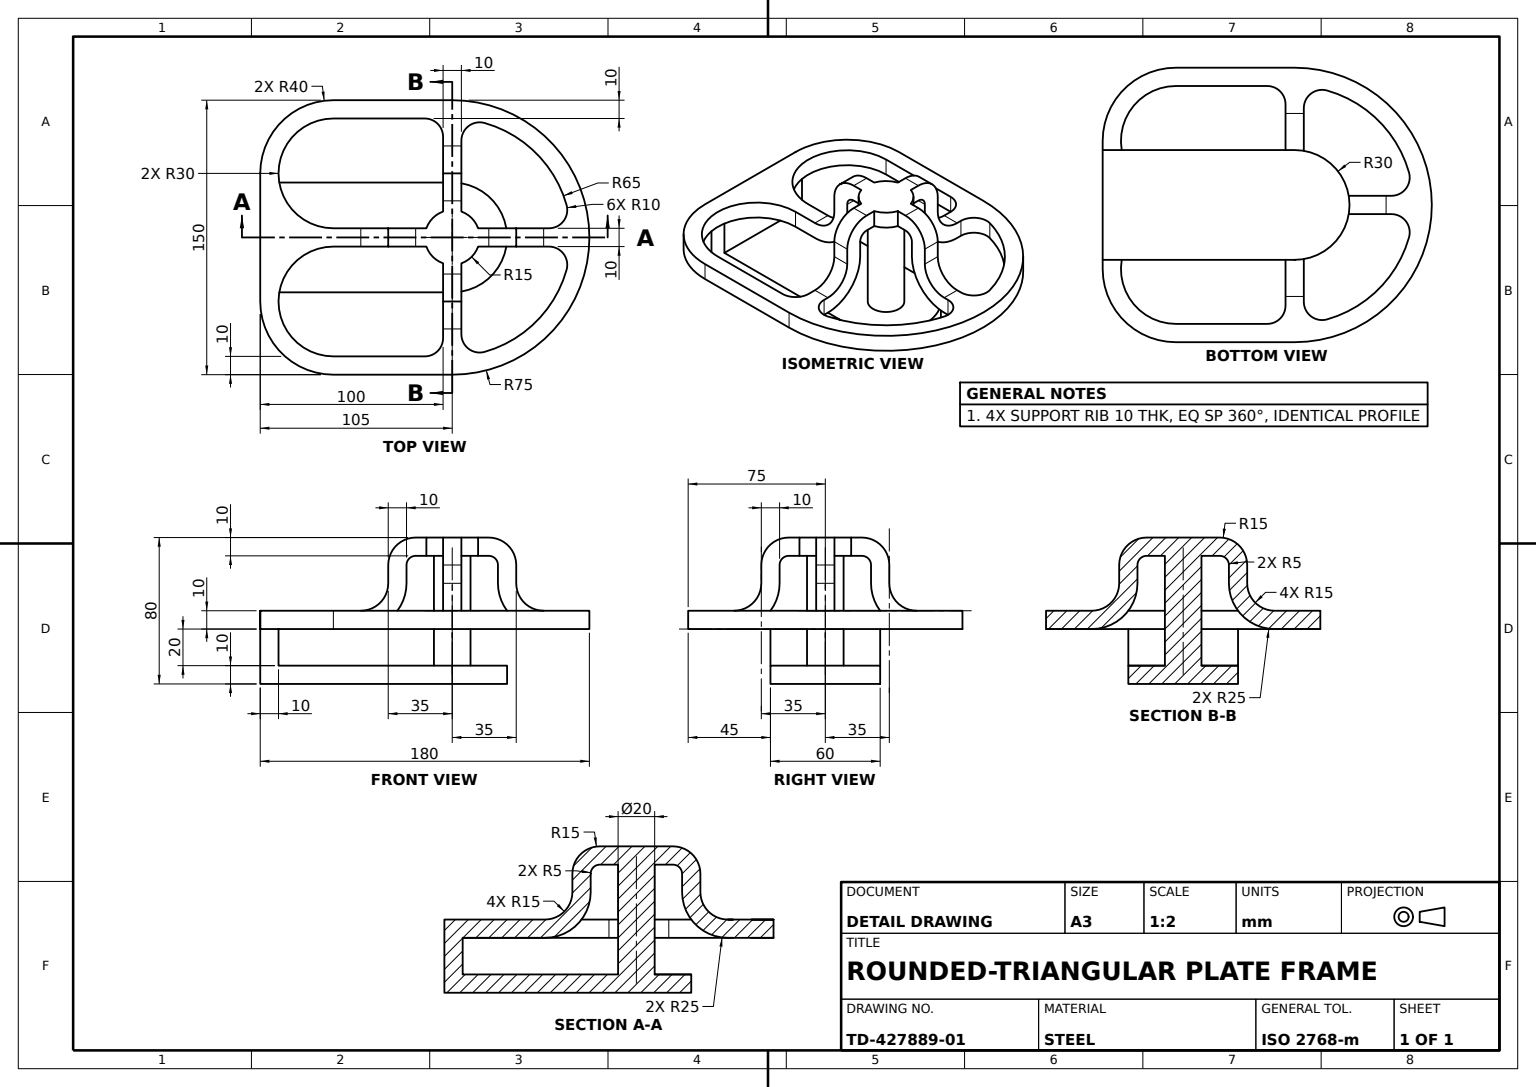
solid
v1 (-95,-30,30)
v2 (-95,-10,30)
e1 v1 v2 LINE
v3 (-105,-10,30)
e2 v2 v3 LINE
v4 (-105,-40,30)
e3 v3 v4 LINE
v5 (0,-40,30)
e4 v5 v4 LINE
v6 (0,-30,30)
e5 v6 v5 LINE
e6 v6 v1 LINE
face PLANE(AX(P(-105,-30,30),D(0,0,1),D(1,0,0))) [e1 e2 e3 -e4 -e5 e6]
v7 (-105,-10,35)
e7 v3 v7 LINE
v8 (-105,0,35)
e8 v7 v8 LINE
v9 (-105,0,-35)
e9 v9 v8 LINE
v10 (-105,-10,-35)
e10 v10 v9 LINE
v11 (-105,-10,-30)
e11 v10 v11 LINE
v12 (-105,-40,-30)
e12 v11 v12 LINE
e13 v4 v12 LINE
face PLANE(AX(P(-105,-10,-35),D(-1,0,0),D(0,0,1))) [e7 e8 -e9 -e10 e11 e12 -e13 -e3]
v13 (0,-30,-30)
e14 v13 v6 CIRCLE(AX(P(0,-30,0),D(0,-1,0),D(0,0,1)),30)
v14 (-95,-30,-30)
e15 v14 v13 LINE
e16 v1 v14 LINE
v15 (0,-30,10)
v16 (0,-30,-10)
e17 v15 v16 CIRCLE(AX(P(0,-30,0),D(0,1,0),D(0,0,1)),10)
e18 v16 v15 CIRCLE(AX(P(0,-30,0),D(0,1,0),D(0,0,1)),10)
face PLANE(AX(P(0,-30,0),D(0,1,0),D(0,0,1))) [-e6 -e14 -e15 -e16] [-e17 -e18]
v17 (-20,30,-5)
v18 (-25,25,-5)
e19 v17 v18 CIRCLE(AX(P(-20,25,-5),D(0,0,1),D(1,0,0)),5)
v19 (-20,30,5)
e20 v19 v17 LINE
v20 (-25,25,5)
e21 v19 v20 CIRCLE(AX(P(-20,25,5),D(0,0,1),D(1,0,0)),5)
e22 v20 v18 LINE
face CYL(AX(P(-20,25,5),D(0,0,-1),D(-1,0,0)),5) rev [-e19 -e20 e21 e22]
v21 (0,-40,-30)
e23 v13 v21 LINE
e24 v21 v5 CIRCLE(AX(P(0,-40,0),D(0,-1,0),D(0,0,1)),30)
face CYL(AX(P(0,-30,0),D(0,-1,0),D(0,0,-1)),30) [-e23 e14 e5 -e24]
v22 (14.142136,40,-5)
v23 (14.142136,30,-5)
e25 v22 v23 LINE
v24 (5,30,-14.142136)
e26 v23 v24 CIRCLE(AX(P(0,30,0),D(0,1,0),D(0,0,1)),15)
v25 (5,40,-14.142136)
e27 v25 v24 LINE
e28 v22 v25 CIRCLE(AX(P(0,40,0),D(0,1,0),D(0,0,1)),15)
face CYL(AX(P(0,30,0),D(0,1,0),D(0,0,1)),15) [e25 e26 -e27 -e28]
v26 (-35,15,5)
v27 (-35,15,-5)
e29 v26 v27 LINE
v28 (-35,25,5)
e30 v28 v26 LINE
v29 (-35,25,-5)
e31 v28 v29 LINE
e32 v29 v27 LINE
face PLANE(AX(P(-35,25,5),D(1,0,0),D(0,1,0))) rev [-e29 -e30 e31 e32]
v30 (5,25,25)
v31 (-5,25,25)
e33 v30 v31 LINE
v32 (5,15,25)
e34 v30 v32 LINE
v33 (-5,15,25)
e35 v32 v33 LINE
e36 v31 v33 LINE
face PLANE(AX(P(5,25,25),D(0,0,-1),D(-1,0,0))) [-e33 e34 e35 -e36]
v34 (20,40,-5)
e37 v22 v34 LINE
v35 (35,25,-5)
e38 v34 v35 CIRCLE(AX(P(20,25,-5),D(0,0,-1),D(-1,0,0)),15)
v36 (35,15,-5)
e39 v35 v36 LINE
v37 (50,0,-5)
e40 v36 v37 CIRCLE(AX(P(50,15,-5),D(0,0,1),D(1,0,0)),15)
v38 (52.915026,0,-5)
e41 v37 v38 LINE
v39 (52.915026,-10,-5)
e42 v39 v38 LINE
v40 (50,-10,-5)
e43 v39 v40 LINE
v41 (25,15,-5)
e44 v41 v40 CIRCLE(AX(P(50,15,-5),D(0,0,1),D(1,0,0)),25)
v42 (25,25,-5)
e45 v42 v41 LINE
v43 (20,30,-5)
e46 v43 v42 CIRCLE(AX(P(20,25,-5),D(0,0,-1),D(-1,0,0)),5)
e47 v23 v43 LINE
face PLANE(AX(P(50,15,-5),D(0,0,1),D(1,0,0))) rev [e37 e38 e39 e40 e41 -e42 e43 -e44 -e45 -e46 -e47 -e25]
v44 (5,40,-20)
v45 (5,25,-35)
e48 v44 v45 CIRCLE(AX(P(5,25,-20),D(-1,0,0),D(0,0,1)),15)
v46 (-5,25,-35)
e49 v46 v45 LINE
v47 (-5,40,-20)
e50 v47 v46 CIRCLE(AX(P(-5,25,-20),D(-1,0,0),D(0,0,1)),15)
e51 v47 v44 LINE
face CYL(AX(P(-5,25,-20),D(1,0,0),D(0,0,-1)),15) [e48 -e49 -e50 e51]
v48 (-5,30,-14.142136)
v49 (-5,40,-14.142136)
e52 v48 v49 LINE
v50 (-14.142136,30,-5)
e53 v48 v50 CIRCLE(AX(P(0,30,0),D(0,1,0),D(0,0,1)),15)
v51 (-14.142136,40,-5)
e54 v51 v50 LINE
e55 v49 v51 CIRCLE(AX(P(0,40,0),D(0,1,0),D(0,0,1)),15)
face CYL(AX(P(0,30,0),D(0,1,0),D(0,0,1)),15) [-e52 e53 -e54 -e55]
v52 (25,15,5)
v53 (50,-10,5)
e56 v52 v53 CIRCLE(AX(P(50,15,5),D(0,0,1),D(1,0,0)),25)
e57 v41 v52 LINE
e58 v40 v53 LINE
face CYL(AX(P(50,15,-5),D(0,0,1),D(1,0,0)),25) [-e56 -e57 e44 e58]
v54 (0,30,-10)
v55 (0,30,10)
e59 v54 v55 CIRCLE(AX(P(0,30,0),D(0,1,0),D(0,0,1)),10)
e60 v54 v16 LINE
e61 v55 v15 LINE
face CYL(AX(P(0,40,0),D(0,-1,0),D(0,0,-1)),10) [-e59 e60 e18 -e61]
v56 (-5,40,14.142136)
v57 (-5,30,14.142136)
e62 v56 v57 LINE
v58 (-14.142136,40,5)
e63 v58 v56 CIRCLE(AX(P(0,40,0),D(0,1,0),D(0,0,1)),15)
v59 (-14.142136,30,5)
e64 v58 v59 LINE
e65 v59 v57 CIRCLE(AX(P(0,30,0),D(0,1,0),D(0,0,1)),15)
face CYL(AX(P(0,30,0),D(0,1,0),D(0,0,1)),15) [-e62 -e63 e64 e65]
v60 (5,-10,50)
e66 v32 v60 CIRCLE(AX(P(5,15,50),D(-1,0,0),D(0,0,1)),25)
v61 (-5,-10,50)
e67 v61 v60 LINE
e68 v33 v61 CIRCLE(AX(P(-5,15,50),D(-1,0,0),D(0,0,1)),25)
face CYL(AX(P(5,15,50),D(-1,0,0),D(0,0,1)),25) [-e35 e66 -e67 -e68]
v62 (0,-10,-75)
v63 (0,0,-75)
e69 v62 v63 LINE
v64 (0,0,75)
e70 v64 v63 CIRCLE(AX(P(0,0,0),D(0,1,0),D(0,0,1)),75)
v65 (0,-10,75)
e71 v65 v64 LINE
e72 v65 v62 CIRCLE(AX(P(0,-10,0),D(0,1,0),D(0,0,1)),75)
face CYL(AX(P(0,-10,0),D(0,1,0),D(0,0,1)),75) [e69 -e70 -e71 e72]
v66 (-5,0,50)
v67 (-5,0,55)
e73 v66 v67 LINE
v68 (-5,15,35)
e74 v68 v66 CIRCLE(AX(P(-5,15,50),D(-1,0,0),D(0,0,1)),15)
v69 (-5,25,35)
e75 v69 v68 LINE
v70 (-5,40,20)
e76 v70 v69 CIRCLE(AX(P(-5,25,20),D(1,0,0),D(0,0,-1)),15)
e77 v56 v70 LINE
v71 (-5,30,20)
e78 v57 v71 LINE
e79 v71 v31 CIRCLE(AX(P(-5,25,20),D(1,0,0),D(0,0,-1)),5)
v72 (-5,-10,55)
e80 v61 v72 LINE
e81 v72 v67 LINE
face PLANE(AX(P(-5,-10,0),D(-1,0,0),D(0,0,1))) [-e73 -e74 -e75 -e76 -e77 e62 e78 e79 e36 e68 e80 e81]
v73 (-65,-10,75)
e82 v73 v65 LINE
v74 (-65,0,75)
e83 v74 v64 LINE
e84 v73 v74 LINE
face PLANE(AX(P(-65,-10,75),D(0,0,1),D(1,0,0))) [e82 e71 -e83 -e84]
v75 (-65,0,5)
v76 (-65,0,65)
e85 v75 v76 CIRCLE(AX(P(-65,0,35),D(0,1,0),D(0,0,1)),30)
v77 (-65,-10,65)
e86 v77 v76 LINE
v78 (-65,-10,5)
e87 v78 v77 CIRCLE(AX(P(-65,-10,35),D(0,1,0),D(0,0,1)),30)
e88 v78 v75 LINE
face CYL(AX(P(-65,-10,35),D(0,1,0),D(0,0,1)),30) rev [e85 -e86 -e87 e88]
v79 (62.53594,-10,-17.727273)
e89 v39 v79 CIRCLE(AX(P(52.915026,-10,-15),D(0,1,0),D(0,0,1)),10)
v80 (62.53594,0,-17.727273)
e90 v38 v80 CIRCLE(AX(P(52.915026,0,-15),D(0,1,0),D(0,0,1)),10)
e91 v79 v80 LINE
face CYL(AX(P(52.915026,-10,-15),D(0,1,0),D(0,0,1)),10) rev [-e89 e42 e90 -e91]
v81 (-5,25,-25)
v82 (-5,15,-25)
e92 v81 v82 LINE
v83 (5,15,-25)
e93 v82 v83 LINE
v84 (5,25,-25)
e94 v84 v83 LINE
e95 v81 v84 LINE
face PLANE(AX(P(-5,25,-25),D(0,0,1),D(1,0,0))) [e92 e93 -e94 -e95]
v85 (17.727273,0,-62.53594)
e96 v80 v85 CIRCLE(AX(P(0,0,0),D(0,1,0),D(0,0,1)),65)
v86 (17.727273,-10,-62.53594)
e97 v86 v85 LINE
e98 v79 v86 CIRCLE(AX(P(0,-10,0),D(0,1,0),D(0,0,1)),65)
face CYL(AX(P(0,-10,0),D(0,1,0),D(0,0,1)),65) rev [e96 -e97 -e98 e91]
v87 (5,15,-35)
e99 v45 v87 LINE
v88 (-5,15,-35)
e100 v88 v87 LINE
e101 v46 v88 LINE
face PLANE(AX(P(-5,25,-35),D(0,0,1),D(1,0,0))) rev [e99 -e100 -e101 e49]
v89 (5,30,-20)
e102 v89 v84 CIRCLE(AX(P(5,25,-20),D(-1,0,0),D(0,0,1)),5)
v90 (5,-10,-50)
e103 v83 v90 CIRCLE(AX(P(5,15,-50),D(1,0,0),D(0,0,-1)),25)
v91 (5,-10,-52.915026)
e104 v91 v90 LINE
v92 (5,0,-52.915026)
e105 v91 v92 LINE
v93 (5,0,-50)
e106 v92 v93 LINE
e107 v87 v93 CIRCLE(AX(P(5,15,-50),D(1,0,0),D(0,0,-1)),15)
e108 v25 v44 LINE
e109 v24 v89 LINE
face PLANE(AX(P(5,-10,0),D(-1,0,0),D(0,0,1))) rev [e102 e94 e103 -e104 e105 e106 -e107 -e99 -e48 -e108 e27 e109]
v94 (15,-10,62.915026)
v95 (17.727273,-10,62.53594)
e110 v94 v95 CIRCLE(AX(P(15,-10,52.915026),D(0,1,0),D(0,0,1)),10)
v96 (15,0,62.915026)
e111 v94 v96 LINE
v97 (17.727273,0,62.53594)
e112 v96 v97 CIRCLE(AX(P(15,0,52.915026),D(0,1,0),D(0,0,1)),10)
e113 v95 v97 LINE
face CYL(AX(P(15,-10,52.915026),D(0,1,0),D(0,0,1)),10) rev [-e110 e111 e112 -e113]
e114 v12 v21 LINE
face PLANE(AX(P(0,-40,0),D(0,1,0),D(0,0,1))) rev [e4 e13 e114 e24]
v98 (-25,15,-5)
v99 (-50,-10,-5)
e115 v98 v99 CIRCLE(AX(P(-50,15,-5),D(0,0,-1),D(-1,0,0)),25)
v100 (-25,15,5)
e116 v100 v98 LINE
v101 (-50,-10,5)
e117 v100 v101 CIRCLE(AX(P(-50,15,5),D(0,0,-1),D(-1,0,0)),25)
e118 v101 v99 LINE
face CYL(AX(P(-50,15,5),D(0,0,-1),D(-1,0,0)),25) [-e115 -e116 e117 e118]
v102 (-5,-10,-50)
e119 v102 v90 LINE
e120 v82 v102 CIRCLE(AX(P(-5,15,-50),D(1,0,0),D(0,0,-1)),25)
face CYL(AX(P(-5,15,-50),D(1,0,0),D(0,0,-1)),25) [e119 -e103 -e93 e120]
v103 (35,25,5)
v104 (35,15,5)
e121 v103 v104 LINE
v105 (20,40,5)
e122 v105 v103 CIRCLE(AX(P(20,25,5),D(0,0,-1),D(-1,0,0)),15)
v106 (14.142136,40,5)
e123 v106 v105 LINE
v107 (14.142136,30,5)
e124 v106 v107 LINE
v108 (20,30,5)
e125 v107 v108 LINE
v109 (25,25,5)
e126 v108 v109 CIRCLE(AX(P(20,25,5),D(0,0,-1),D(-1,0,0)),5)
e127 v109 v52 LINE
v110 (52.915026,-10,5)
e128 v110 v53 LINE
v111 (52.915026,0,5)
e129 v110 v111 LINE
v112 (50,0,5)
e130 v112 v111 LINE
e131 v104 v112 CIRCLE(AX(P(50,15,5),D(0,0,1),D(1,0,0)),15)
face PLANE(AX(P(50,15,5),D(0,0,1),D(1,0,0))) [-e121 -e122 -e123 e124 e125 e126 e127 e56 -e128 e129 -e130 -e131]
v113 (-15,-10,65)
v114 (-15,0,65)
e132 v113 v114 LINE
e133 v67 v114 CIRCLE(AX(P(-15,0,55),D(0,-1,0),D(0,0,1)),10)
e134 v72 v113 CIRCLE(AX(P(-15,-10,55),D(0,-1,0),D(0,0,1)),10)
face CYL(AX(P(-15,-10,55),D(0,1,0),D(0,0,1)),10) rev [e132 -e133 -e81 e134]
v115 (-65,-10,-75)
e135 v62 v115 LINE
v116 (-65,0,-75)
e136 v115 v116 LINE
e137 v63 v116 LINE
face PLANE(AX(P(-65,-10,-75),D(0,0,-1),D(-1,0,0))) [e135 e136 -e137 -e69]
v117 (-20,40,-5)
e138 v51 v117 LINE
e139 v50 v17 LINE
e140 v18 v98 LINE
v118 (-65,-10,-5)
e141 v118 v99 LINE
v119 (-65,0,-5)
e142 v118 v119 LINE
v120 (-50,0,-5)
e143 v120 v119 LINE
e144 v27 v120 CIRCLE(AX(P(-50,15,-5),D(0,0,-1),D(-1,0,0)),15)
e145 v117 v29 CIRCLE(AX(P(-20,25,-5),D(0,0,1),D(1,0,0)),15)
face PLANE(AX(P(-50,15,-5),D(0,0,-1),D(-1,0,0))) [-e138 e54 e139 e19 e140 e115 -e141 e142 -e143 -e144 -e32 -e145]
v121 (-5,-10,-55)
e146 v121 v102 LINE
v122 (-5,30,-20)
e147 v122 v81 CIRCLE(AX(P(-5,25,-20),D(-1,0,0),D(0,0,1)),5)
e148 v122 v48 LINE
e149 v47 v49 LINE
v123 (-5,0,-50)
e150 v88 v123 CIRCLE(AX(P(-5,15,-50),D(1,0,0),D(0,0,-1)),15)
v124 (-5,0,-55)
e151 v124 v123 LINE
e152 v121 v124 LINE
face PLANE(AX(P(-5,-10,0),D(-1,0,0),D(0,0,1))) [e146 -e120 -e92 -e147 e148 e52 -e149 e50 e101 e150 -e151 -e152]
v125 (-50,0,5)
e153 v125 v120 LINE
e154 v26 v125 CIRCLE(AX(P(-50,15,5),D(0,0,-1),D(-1,0,0)),15)
face CYL(AX(P(-50,15,5),D(0,0,-1),D(-1,0,0)),15) rev [e29 e144 -e153 -e154]
v126 (-95,-10,-30)
e155 v14 v126 LINE
e156 v126 v11 LINE
face PLANE(AX(P(-105,-30,-30),D(0,0,-1),D(-1,0,0))) [-e155 e15 e23 -e114 -e12 -e156]
v127 (5,15,35)
v128 (5,0,50)
e157 v127 v128 CIRCLE(AX(P(5,15,50),D(-1,0,0),D(0,0,1)),15)
e158 v127 v68 LINE
e159 v66 v128 LINE
face CYL(AX(P(5,15,50),D(-1,0,0),D(0,0,1)),15) rev [-e157 e158 e74 e159]
v129 (62.53594,-10,17.727273)
e160 v110 v129 CIRCLE(AX(P(52.915026,-10,15),D(0,-1,0),D(0,0,1)),10)
v130 (62.53594,0,17.727273)
e161 v129 v130 LINE
e162 v111 v130 CIRCLE(AX(P(52.915026,0,15),D(0,-1,0),D(0,0,1)),10)
face CYL(AX(P(52.915026,-10,15),D(0,1,0),D(0,0,1)),10) rev [e160 e161 -e162 -e129]
v131 (5,40,14.142136)
e163 v131 v106 CIRCLE(AX(P(0,40,0),D(0,1,0),D(0,0,1)),15)
v132 (5,30,14.142136)
e164 v131 v132 LINE
e165 v132 v107 CIRCLE(AX(P(0,30,0),D(0,1,0),D(0,0,1)),15)
face CYL(AX(P(0,30,0),D(0,1,0),D(0,0,1)),15) [-e163 e164 e165 -e124]
e166 v36 v104 LINE
e167 v35 v103 LINE
face PLANE(AX(P(35,25,-5),D(-1,0,0),D(0,-1,0))) rev [e121 -e166 -e39 e167]
v133 (-65,-10,-65)
e168 v133 v118 CIRCLE(AX(P(-65,-10,-35),D(0,1,0),D(0,0,1)),30)
v134 (-65,0,-65)
e169 v133 v134 LINE
e170 v134 v119 CIRCLE(AX(P(-65,0,-35),D(0,1,0),D(0,0,1)),30)
face CYL(AX(P(-65,-10,-35),D(0,1,0),D(0,0,1)),30) rev [-e142 -e168 e169 e170]
e171 v20 v100 LINE
face PLANE(AX(P(-25,25,5),D(1,0,0),D(0,0,-1))) [e116 -e140 -e22 e171]
e172 v123 v93 LINE
face CYL(AX(P(-5,15,-50),D(1,0,0),D(0,0,-1)),15) rev [-e172 -e150 e100 e107]
e173 v55 v54 CIRCLE(AX(P(0,30,0),D(0,1,0),D(0,0,1)),10)
e174 v122 v89 LINE
e175 v43 v108 LINE
v135 (5,30,20)
e176 v132 v135 LINE
e177 v135 v71 LINE
e178 v59 v19 LINE
face PLANE(AX(P(0,30,0),D(0,1,0),D(0,0,1))) rev [e59 e173] [e20 -e139 -e53 -e148 e174 -e109 -e26 e47 e175 -e125 -e165 e176 e177 -e78 -e65 e178]
e179 v34 v105 LINE
v136 (-20,40,5)
e180 v136 v117 LINE
e181 v58 v136 LINE
v137 (5,40,20)
e182 v137 v70 LINE
e183 v131 v137 LINE
face PLANE(AX(P(0,40,0),D(0,1,0),D(0,0,1))) [e123 -e179 -e37 e28 e108 -e51 e149 e55 e138 -e180 -e181 e63 e77 -e182 -e183 e163]
v138 (-15,-10,-65)
e184 v121 v138 CIRCLE(AX(P(-15,-10,-55),D(0,1,0),D(0,0,1)),10)
e185 v138 v133 LINE
e186 v78 v101 LINE
e187 v77 v113 LINE
v139 (5,-10,52.915026)
e188 v60 v139 LINE
e189 v139 v94 CIRCLE(AX(P(15,-10,52.915026),D(0,1,0),D(0,0,1)),10)
e190 v95 v129 CIRCLE(AX(P(0,-10,0),D(0,1,0),D(0,0,1)),65)
e191 v86 v91 CIRCLE(AX(P(15,-10,-52.915026),D(0,1,0),D(0,0,1)),10)
e192 v7 v73 CIRCLE(AX(P(-65,-10,35),D(0,1,0),D(0,0,-1)),40)
e193 v2 v126 LINE
e194 v115 v10 CIRCLE(AX(P(-65,-10,-35),D(0,1,0),D(0,0,-1)),40)
face PLANE(AX(P(-65,-10,35),D(0,-1,0),D(0,0,-1))) [e104 -e119 -e146 e184 e185 e168 e141 -e118 -e186 e87 e187 -e134 -e80 e67 e188 e189 e110 e190 -e160 e128 -e58 -e43 e89 e98 e191] [-e82 -e192 -e7 -e2 e193 e156 -e11 -e194 -e135 -e72]
face CYL(AX(P(20,25,-5),D(0,0,1),D(1,0,0)),15) [e122 -e167 -e38 e179]
e195 v8 v74 CIRCLE(AX(P(-65,0,35),D(0,1,0),D(0,0,-1)),40)
face CYL(AX(P(-65,-10,35),D(0,1,0),D(0,0,1)),40) [-e195 -e8 e192 e84]
e196 v37 v112 LINE
face CYL(AX(P(50,15,-5),D(0,0,1),D(1,0,0)),15) rev [e131 -e196 -e40 e166]
e197 v85 v92 CIRCLE(AX(P(15,0,-52.915026),D(0,1,0),D(0,0,1)),10)
face CYL(AX(P(15,-10,-52.915026),D(0,1,0),D(0,0,1)),10) rev [e97 e197 -e105 -e191]
e198 v97 v130 CIRCLE(AX(P(0,0,0),D(0,1,0),D(0,0,1)),65)
face CYL(AX(P(0,-10,0),D(0,1,0),D(0,0,1)),65) rev [e113 e198 -e161 -e190]
face CYL(AX(P(0,40,0),D(0,-1,0),D(0,0,-1)),10) [e61 e17 -e60 -e173]
v140 (-15,0,-65)
e199 v124 v140 CIRCLE(AX(P(-15,0,-55),D(0,1,0),D(0,0,1)),10)
e200 v138 v140 LINE
face CYL(AX(P(-15,-10,-55),D(0,1,0),D(0,0,1)),10) rev [e152 e199 -e200 -e184]
e201 v42 v109 LINE
face PLANE(AX(P(25,25,-5),D(-1,0,0),D(0,0,1))) [e45 e57 -e127 -e201]
e202 v140 v134 LINE
face PLANE(AX(P(0,-10,-65),D(0,0,-1),D(-1,0,0))) rev [-e185 e200 e202 -e169]
v141 (5,25,35)
e203 v141 v127 LINE
e204 v141 v69 LINE
face PLANE(AX(P(5,25,35),D(0,0,-1),D(-1,0,0))) rev [-e203 e204 e75 -e158]
e205 v76 v114 LINE
face PLANE(AX(P(0,-10,65),D(0,0,1),D(1,0,0))) rev [-e187 e86 e205 -e132]
e206 v135 v30 CIRCLE(AX(P(5,25,20),D(1,0,0),D(0,0,-1)),5)
e207 v137 v141 CIRCLE(AX(P(5,25,20),D(1,0,0),D(0,0,-1)),15)
v142 (5,0,52.915026)
e208 v128 v142 LINE
e209 v139 v142 LINE
face PLANE(AX(P(5,-10,0),D(-1,0,0),D(0,0,1))) rev [-e188 -e66 -e34 -e206 -e176 -e164 e183 e207 e203 e157 e208 -e209]
face CYL(AX(P(20,25,-5),D(0,0,1),D(1,0,0)),5) rev [-e126 -e175 e46 e201]
face CYL(AX(P(-5,25,-20),D(1,0,0),D(0,0,-1)),5) rev [e95 -e102 -e174 e147]
e210 v136 v28 CIRCLE(AX(P(-20,25,5),D(0,0,1),D(1,0,0)),15)
face CYL(AX(P(-20,25,5),D(0,0,-1),D(-1,0,0)),15) [-e210 e180 e145 -e31]
face CYL(AX(P(5,25,20),D(-1,0,0),D(0,0,1)),15) [-e207 e182 e76 -e204]
e211 v116 v9 CIRCLE(AX(P(-65,0,-35),D(0,1,0),D(0,0,-1)),40)
face CYL(AX(P(-65,-10,-35),D(0,1,0),D(0,0,1)),40) [e194 e10 -e211 -e136]
e212 v142 v96 CIRCLE(AX(P(15,0,52.915026),D(0,1,0),D(0,0,1)),10)
face CYL(AX(P(15,-10,52.915026),D(0,1,0),D(0,0,1)),10) rev [-e111 -e189 e209 e212]
e213 v125 v75 LINE
face PLANE(AX(P(-65,0,35),D(0,-1,0),D(0,0,-1))) rev [-e202 -e199 e151 e172 -e106 -e197 -e96 -e90 -e41 e196 e130 e162 -e198 -e112 -e212 -e208 -e159 e73 e133 -e205 -e85 -e213 e153 e143 -e170] [e83 e70 e137 e211 e9 e195]
face CYL(AX(P(5,25,20),D(-1,0,0),D(0,0,1)),5) rev [-e177 e206 e33 -e79]
face PLANE(AX(P(-95,-10,30),D(-1,0,0),D(0,0,1))) rev [e155 -e193 -e1 e16]
face PLANE(AX(P(-50,15,5),D(0,0,-1),D(-1,0,0))) rev [e213 -e88 e186 -e117 -e171 -e21 -e178 -e64 e181 e210 e30 e154]
